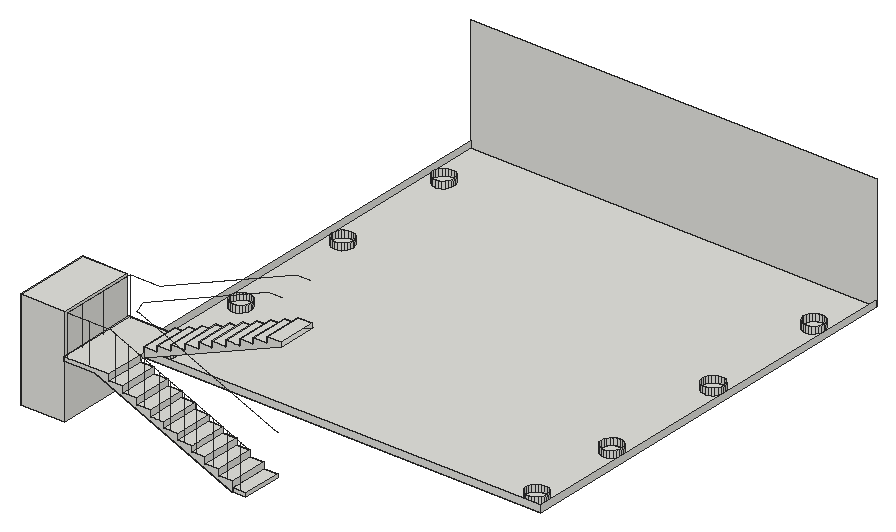
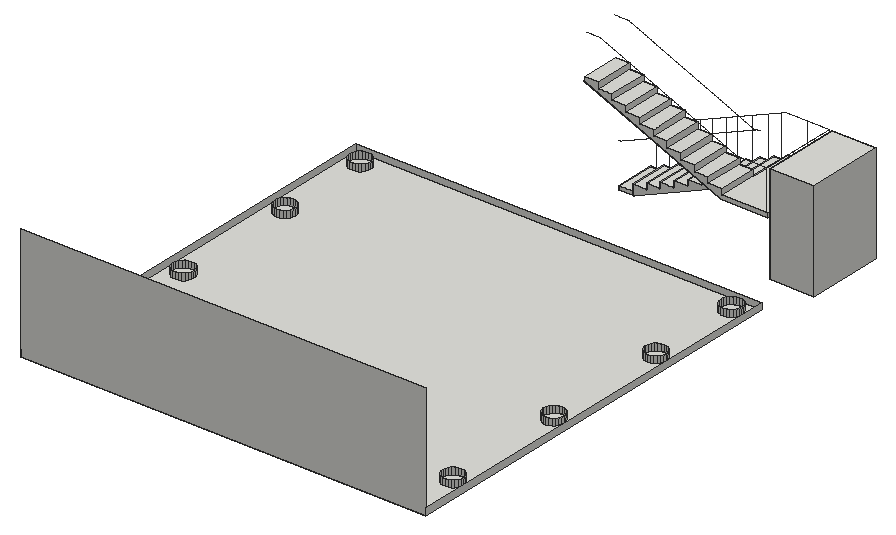
# SketchUp Ruby script. Lengths in millimetres.
U = 1.mm
M = Sketchup.active_model
def pt(a) = Geom::Point3d.new(a.map { |v| v * U })
def face(e, loops, mat)
  f = e.add_face(loops[0].map { |a| pt(a) })
  loops[1..].each { |l| e.add_face(l.map { |a| pt(a) }).erase! }
  f.material = f.back_material = mat if mat
  f
end
# faces: each face lists its corners as indices into pts; further lists are holes
def faces(e, pts, list, mat = nil) = list.each { |f| face(e, (f[0].is_a?(Array) ? f : [f]).map { |l| l.map { |i| pts[i] } }, mat) }
# xy, xz, yz: faces in a plane at the given z, y or x. An outline is a flat list of corners, or four numbers for a rectangle; further outlines are holes
def ring(l) = l.size == 4 ? [[l[0], l[1]], [l[2], l[1]], [l[2], l[3]], [l[0], l[3]]] : l.each_slice(2).to_a
def flat(e, list, mat, &to3) = list.each { |f| face(e, (f[0].is_a?(Array) ? f : [f]).map { |l| ring(l).map { |u, v| to3.(u, v) } }, mat) }
def xy(e, z, list, mat = nil) = flat(e, list, mat) { |x, y| [x, y, z] }
def xz(e, y, list, mat = nil) = flat(e, list, mat) { |x, z| [x, y, z] }
def yz(e, x, list, mat = nil) = flat(e, list, mat) { |y, z| [x, y, z] }
def lines(e, pts, list) = list.each { |a, b| e.add_line(pt(pts[a]), pt(pts[b])) }
# prism: a flat outline (further loops are holes) pulled along v
def prism(e, loops, v, mat = nil)
  f = face(e, loops, mat); d = Geom::Vector3d.new(v.map { |x| x * U })
  f.pushpull(f.normal.samedirection?(d) ? d.length : -d.length)
end
def box(e, o, s, mat = nil) = prism(e, [[o, [o[0] + s[0], o[1], o[2]], [o[0] + s[0], o[1] + s[1], o[2]], [o[0], o[1] + s[1], o[2]]]], [0, 0, s[2]], mat)
def at(x, y, z, deg = 0) = Geom::Transformation.translation(pt([x, y, z])) * Geom::Transformation.rotation(ORIGIN, Z_AXIS, deg.degrees)
def axes(o, x, y, z) = Geom::Transformation.new([*x, 0, *y, 0, *z, 0, *pt(o).to_a, 1])
def part(name) = M.definitions.add(name)
# library, detail: a bought-in or finely detailed component or shape, given as its bounding box
def library(name, o, s) = part(name).tap { |d| box(d.entities, o, s) }
def detail(e, o, s) = box(e.add_group.entities, o, s)
def put(e, d, t, mat = nil) = e.add_instance(d, t).tap { |i| i.material = mat if mat }
def group(e, t, mat = nil) = e.add_group.tap { |g| g.transformation = t; g.material = mat if mat }.entities
root = M.entities
c1 = part("Group55\#2")
p = [[13622.3,-331.8,4572],[13622.3,-282.6,4572],[13622.3,2717.8,6064.2],[13622.3,3668.7,6064.2],[15624.2,3668.7,6064.2],[15624.2,3017.8,6064.2],
  [15624.2,17.5,7556.5],[15624.2,-282.6,7556.5],[14524,-331.8,4572],[14524,-282.6,4572],[14524,2717.8,6064.2],[14524,2767,6064.2],
  [14722.5,2767,6189],[14722.5,17.5,7556.5],[14722.5,-282.6,7556.5]]
lines(c1.entities,p,[[0,1],[1,2],[2,3],[3,4],[4,5],[5,6],[6,7],[8,9],[9,10],[10,11],[11,12],[12,13],
  [13,14]])
c2 = part("Group54\#1")
xy(c2.entities,4472,[[13573.1,-282.6,14573.2,17.5],[13573.1,17.5,14573.2,41]])
xy(c2.entities,4572,[[13573.1,-282.6,14573.2,17.5]])
xy(c2.entities,4721.2,[[13573.1,17.5,14573.2,317.5]])
xy(c2.entities,4870.4,[[13573.1,317.5,14573.2,617.5]])
xy(c2.entities,5019.7,[[13573.1,617.5,14573.2,617.5,14573.3,917.6,13573.1,917.6]])
xy(c2.entities,5168.9,[[13573.1,917.6,14573.3,917.6,14573.2,1217.6,13573.1,1217.6]])
xy(c2.entities,5318.1,[[13573.1,1217.6,14573.2,1517.7]])
xy(c2.entities,5467.3,[[13573.1,1517.7,14573.2,1817.7]])
xy(c2.entities,5616.6,[[13573.1,1817.7,14573.2,2117.7]])
xy(c2.entities,5765.8,[[13573.1,2117.7,14573.2,2417.8]])
xy(c2.entities,5915,[[13573.1,2417.8,14573.2,2717.8]])
xy(c2.entities,5964.2,[[14673.3,2694.3,14673.3,2717.8,14573.2,2717.8,14573.2,3041.3,13573.1,3041.3,13573.1,3717.9,15673.4,3717.9,15673.4,2694.3]])
xy(c2.entities,6064.2,[[13573.1,2717.8,15673.4,3717.9]])
xy(c2.entities,6213.5,[[14673.3,2417.8,15673.4,2717.8]])
xy(c2.entities,6362.7,[[14673.3,2117.7,15673.4,2417.8]])
xy(c2.entities,6511.9,[[14673.3,1817.7,15673.4,2117.7]])
xy(c2.entities,6661.1,[[14673.3,1517.7,15673.4,1817.7]])
xy(c2.entities,6810.4,[[14673.3,1217.6,15673.4,1517.7]])
xy(c2.entities,6959.6,[[14673.3,917.6,15673.4,1217.6]])
xy(c2.entities,7108.8,[[14673.3,617.5,15673.4,917.6]])
xy(c2.entities,7258,[[14673.3,317.5,15673.4,617.5]])
xy(c2.entities,7407.3,[[14673.3,17.5,15673.4,317.5]])
xy(c2.entities,7556.5,[[14673.3,-282.6,15673.4,17.5]])
xz(c2.entities,-282.6,[[13573.1,4472,14573.2,4572]])
xz(c2.entities,17.5,[[13573.1,4472,14573.2,4572],[13573.1,4572,14573.2,4721.2],[14673.3,7407.3,15673.4,7556.5]])
xz(c2.entities,317.5,[[13573.1,4721.2,14573.2,4870.4],[14673.3,7258,15673.4,7407.3]])
xz(c2.entities,617.5,[[13573.1,4870.4,14573.2,5019.7],[14673.3,7108.8,15673.4,7258]])
xz(c2.entities,917.6,[[13573.1,5019.7,14573.3,5168.9],[14673.3,6959.6,15673.4,7108.8]])
xz(c2.entities,1217.6,[[13573.1,5168.9,14573.2,5318.1],[14673.3,6810.4,15673.4,6959.6]])
xz(c2.entities,1517.7,[[13573.1,5318.1,14573.2,5467.3],[14673.3,6661.1,15673.4,6810.4]])
xz(c2.entities,1817.7,[[13573.1,5467.3,14573.2,5616.6],[14673.3,6511.9,15673.4,6661.1]])
xz(c2.entities,2117.7,[[13573.1,5616.6,14573.2,5765.8],[14673.3,6362.7,15673.4,6511.9]])
xz(c2.entities,2417.8,[[13573.1,5765.8,14573.2,5915],[14673.3,6213.5,15673.4,6362.7]])
xz(c2.entities,2717.8,[[13573.1,5915,14573.2,6064.2],[14573.2,5964.2,14673.3,6064.2],[14673.3,6064.2,15673.4,6213.5]])
xz(c2.entities,3717.9,[[13573.1,5964.2,15673.4,6064.2]])
yz(c2.entities,13573.1,[[-282.6,4472,17.5,4572],[17.5,4472,17.5,4721.2,317.5,4721.2,317.5,4870.4,617.5,4870.4,617.5,5019.7,917.6,5019.7,917.6,5168.9,1217.6,5168.9,1217.6,5318.1,1517.7,5318.1,1517.7,5467.3,1817.7,5467.3,1817.7,5616.6,2117.7,5616.6,2117.7,5765.8,2417.8,5765.8,2417.8,5915,2717.8,5915,2717.8,6064.2,3717.9,6064.2,3717.9,5964.2,3041.3,5964.2,41,4472]])
yz(c2.entities,14573.2,[[-282.6,4472,17.5,4572]])
yz(c2.entities,14673.3,[[2694.3,5964.2,-306.1,7456.5,-282.6,7456.5,-282.6,7556.5,17.5,7556.5,17.5,7407.3,317.5,7407.3,317.5,7258,617.5,7258,617.5,7108.8,917.6,7108.8,917.6,6959.6,1217.6,6959.6,1217.6,6810.4,1517.7,6810.4,1517.7,6661.1,1817.7,6661.1,1817.7,6511.9,2117.7,6511.9,2117.7,6362.7,2417.8,6362.7,2417.8,6213.5,2717.8,6213.5,2717.8,5964.2]])
yz(c2.entities,15673.4,[[2694.3,5964.2,3717.9,5964.2,3717.9,6064.2,2717.8,6064.2,2717.8,6213.5,2417.8,6213.5,2417.8,6362.7,2117.7,6362.7,2117.7,6511.9,1817.7,6511.9,1817.7,6661.1,1517.7,6661.1,1517.7,6810.4,1217.6,6810.4,1217.6,6959.6,917.6,6959.6,917.6,7108.8,617.5,7108.8,617.5,7258,317.5,7258,317.5,7407.3,17.5,7407.3,17.5,7556.5,-282.6,7556.5,-282.6,7456.5,-306.1,7456.5]])
p = [[14573.2,3041.3,5964.2],[14573.2,2717.8,5964.2],[14573.2,2717.8,5915],[14573.2,2417.8,5915],[14573.2,2417.8,5765.8],[14573.2,2117.7,5765.8],
  [14573.2,2117.7,5616.6],[14573.2,1817.7,5616.6],[14573.2,1817.7,5467.3],[14573.2,1517.7,5467.3],[14573.2,1517.7,5318.1],[14573.2,1217.6,5318.1],
  [14573.2,1217.6,5168.9],[14573.3,917.6,5168.9],[14573.3,917.6,5019.7],[14573.2,617.5,5019.7],[14573.2,617.5,4870.4],[14573.2,317.5,4870.4],
  [14573.2,317.5,4721.2],[14573.2,17.5,4721.2],[14573.2,17.5,4572],[14573.2,17.5,4472],[14573.2,41,4472],[13573.1,41,4472],
  [13573.1,3041.3,5964.2],[15673.4,2694.3,5964.2],[15673.4,-306.1,7456.5],[14673.3,-306.1,7456.5],[14673.3,2694.3,5964.2],[13622.3,3193.3,7064.4],
  [13622.3,3193.3,6064.2],[13622.3,3668.7,7064.4],[13622.3,3668.7,6064.2],[15624.2,3668.7,7064.4],[15624.2,3668.7,6064.2],[14776.1,3668.7,7064.4],
  [14776.1,3668.7,6064.2],[14085.5,3668.7,7064.4],[14085.5,3668.7,6064.2],[13622.3,2628.2,7019.8],[13622.3,2628.2,5915],[13622.3,2338.2,6875.6],
  [13622.3,2338.2,5765.8],[13622.3,1987.6,6701.2],[13622.3,1987.6,5616.6],[13622.3,1654.5,6535.6],[13622.3,1654.5,5467.3],[13622.3,1115.8,6267.6],
  [13622.3,1115.8,5168.9],[13622.3,1403.5,6410.7],[13622.3,1403.5,5318.1],[13622.3,834.6,6127.8],[13622.3,834.6,5019.7],[13622.3,469.4,5946.1],
  [13622.3,469.4,4870.4],[13622.3,173.1,5798.7],[13622.3,173.1,4721.2],[13622.3,-122.5,5651.7],[13622.3,-122.5,4572]]
faces(c2.entities,p,[[0,1,2,3,4,5,6,7,8,9,10,11,12,13,14,15,16,17,18,19,20,21,22],[23,24,0,22],[25,26,27,28]])
lines(c2.entities,p,[[29,30],[31,32],[33,34],[35,36],[37,38],[39,40],[41,42],[43,44],[45,46],[47,48],[49,50],[51,52],
  [53,54],[55,56],[57,58]])
put(c2.entities,c1,at(0,0,1000.1))
xy(root,0,[[[720.2,4710,16417.4,20943.1],[15750.9,18372.1,15853.3,18390.3,15947.6,18434.3,16027.2,18501.2,16086.8,18586.5,16122.3,18684.3,16131.3,18787.9,16113.1,18890.3,16069.1,18984.6,16002.1,19064.2,15916.9,19123.8,15819.1,19159.3,15715.5,19168.3,15613.1,19150.1,15518.8,19106.1,15439.2,19039.1,15379.6,18953.9,15344.1,18856.1,15335.1,18752.5,15353.3,18650.1,15397.3,18555.8,15464.2,18476.2,15549.5,18416.6,15647.3,18381.1],[15768.9,8578.8,15871.3,8597,15965.5,8641,16045.1,8707.9,16104.7,8793.2,16140.2,8891,16149.2,8994.6,16131.1,9097,16087,9191.3,16020.1,9270.9,15934.8,9330.5,15837.1,9366,15733.4,9375,15631,9356.8,15536.8,9312.8,15457.1,9245.9,15397.6,9160.6,15362.1,9062.8,15353.1,8959.2,15371.2,8856.8,15415.3,8762.5,15482.2,8682.9,15567.5,8623.3,15665.2,8587.8],[1429.7,8578.8,1532.1,8597,1626.3,8641,1705.9,8707.9,1765.5,8793.2,1801,8891,1810,8994.6,1791.9,9097,1747.8,9191.3,1680.9,9270.9,1595.6,9330.5,1497.9,9366,1394.2,9375,1291.8,9356.8,1197.6,9312.8,1117.9,9245.9,1058.4,9160.6,1022.9,9062.8,1013.9,8959.2,1032,8856.8,1076.1,8762.5,1143,8682.9,1228.3,8623.3,1326,8587.8],[1429.7,18372.1,1532.1,18390.3,1626.3,18434.3,1705.9,18501.2,1765.5,18586.5,1801,18684.3,1810,18787.9,1791.9,18890.3,1747.8,18984.6,1680.9,19064.2,1595.6,19123.8,1497.9,19159.3,1394.2,19168.3,1291.8,19150.1,1197.6,19106.1,1117.9,19039.1,1058.4,18953.9,1022.9,18856.1,1013.9,18752.5,1032,18650.1,1076.1,18555.8,1143,18476.2,1228.3,18416.6,1326,18381.1],[1429.7,4921.2,1532.1,4939.4,1626.3,4983.4,1705.9,5050.3,1765.5,5135.6,1801,5233.4,1810,5337,1791.9,5439.4,1747.8,5533.7,1680.9,5613.3,1595.6,5672.9,1497.9,5708.4,1394.2,5717.4,1291.8,5699.2,1197.6,5655.2,1117.9,5588.3,1058.4,5503,1022.9,5405.2,1013.9,5301.6,1032,5199.2,1076.1,5104.9,1143,5025.3,1228.3,4965.7,1326,4930.2],[15787,4921.2,15889.4,4939.4,15983.7,4983.4,16063.3,5050.3,16122.9,5135.6,16158.4,5233.4,16167.4,5337,16149.2,5439.4,16105.2,5533.7,16038.3,5613.3,15953,5672.9,15855.2,5708.4,15751.6,5717.4,15649.2,5699.2,15554.9,5655.2,15475.3,5588.3,15415.7,5503,15380.2,5405.2,15371.2,5301.6,15389.4,5199.2,15433.4,5104.9,15500.3,5025.3,15585.6,4965.7,15683.4,4930.2],[15759.9,13504.8,15862.3,13523,15956.5,13567,16036.2,13634,16095.8,13719.2,16131.3,13817,16140.2,13920.6,16122.1,14023,16078.1,14117.3,16011.1,14196.9,15925.9,14256.5,15828.1,14292,15724.5,14301,15622,14282.8,15527.8,14238.8,15448.2,14171.9,15388.6,14086.6,15353.1,13988.8,15344.1,13885.2,15362.2,13782.8,15406.3,13688.5,15473.2,13608.9,15558.5,13549.3,15656.2,13513.8],[1429.7,13504.8,1532.1,13523,1626.3,13567,1705.9,13634,1765.5,13719.2,1801,13817,1810,13920.6,1791.9,14023,1747.8,14117.3,1680.9,14196.9,1595.6,14256.5,1497.9,14292,1394.2,14301,1291.8,14282.8,1197.6,14238.8,1117.9,14171.9,1058.4,14086.6,1022.9,13988.8,1013.9,13885.2,1032,13782.8,1076.1,13688.5,1143,13608.9,1228.3,13549.3,1326,13513.8]],[1429.7,4921.2,1326,4930.2,1228.3,4965.7,1143,5025.3,1076.1,5104.9,1032,5199.2,1013.9,5301.6,1022.9,5405.2,1058.4,5503,1117.9,5588.3,1197.6,5655.2,1291.8,5699.2,1394.2,5717.4,1497.9,5708.4,1595.6,5672.9,1680.9,5613.3,1747.8,5533.7,1791.9,5439.4,1810,5337,1801,5233.4,1765.5,5135.6,1705.9,5050.3,1626.3,4983.4,1532.1,4939.4],[15787,4921.2,15683.4,4930.2,15585.6,4965.7,15500.3,5025.3,15433.4,5104.9,15389.4,5199.2,15371.2,5301.6,15380.2,5405.2,15415.7,5503,15475.3,5588.3,15554.9,5655.2,15649.2,5699.2,15751.6,5717.4,15855.2,5708.4,15953,5672.9,16038.3,5613.3,16105.2,5533.7,16149.2,5439.4,16167.4,5337,16158.4,5233.4,16122.9,5135.6,16063.3,5050.3,15983.7,4983.4,15889.4,4939.4],[1429.7,8578.8,1326,8587.8,1228.3,8623.3,1143,8682.9,1076.1,8762.5,1032,8856.8,1013.9,8959.2,1022.9,9062.8,1058.4,9160.6,1117.9,9245.9,1197.6,9312.8,1291.8,9356.8,1394.2,9375,1497.9,9366,1595.6,9330.5,1680.9,9270.9,1747.8,9191.3,1791.9,9097,1810,8994.6,1801,8891,1765.5,8793.2,1705.9,8707.9,1626.3,8641,1532.1,8597],[15768.9,8578.8,15665.2,8587.8,15567.5,8623.3,15482.2,8682.9,15415.3,8762.5,15371.2,8856.8,15353.1,8959.2,15362.1,9062.8,15397.6,9160.6,15457.1,9245.9,15536.8,9312.8,15631,9356.8,15733.4,9375,15837.1,9366,15934.8,9330.5,16020.1,9270.9,16087,9191.3,16131.1,9097,16149.2,8994.6,16140.2,8891,16104.7,8793.2,16045.1,8707.9,15965.5,8641,15871.3,8597],
  [1429.7,13504.8,1326,13513.8,1228.3,13549.3,1143,13608.9,1076.1,13688.5,1032,13782.8,1013.9,13885.2,1022.9,13988.8,1058.4,14086.6,1117.9,14171.9,1197.6,14238.8,1291.8,14282.8,1394.2,14301,1497.9,14292,1595.6,14256.5,1680.9,14196.9,1747.8,14117.3,1791.9,14023,1810,13920.6,1801,13817,1765.5,13719.2,1705.9,13634,1626.3,13567,1532.1,13523],[15759.9,13504.8,15656.2,13513.8,15558.5,13549.3,15473.2,13608.9,15406.3,13688.5,15362.2,13782.8,15344.1,13885.2,15353.1,13988.8,15388.6,14086.6,15448.2,14171.9,15527.8,14238.8,15622,14282.8,15724.5,14301,15828.1,14292,15925.9,14256.5,16011.1,14196.9,16078.1,14117.3,16122.1,14023,16140.2,13920.6,16131.3,13817,16095.8,13719.2,16036.2,13634,15956.5,13567,15862.3,13523],[1429.7,18372.1,1326,18381.1,1228.3,18416.6,1143,18476.2,1076.1,18555.8,1032,18650.1,1013.9,18752.5,1022.9,18856.1,1058.4,18953.9,1117.9,19039.1,1197.6,19106.1,1291.8,19150.1,1394.2,19168.3,1497.9,19159.3,1595.6,19123.8,1680.9,19064.2,1747.8,18984.6,1791.9,18890.3,1810,18787.9,1801,18684.3,1765.5,18586.5,1705.9,18501.2,1626.3,18434.3,1532.1,18390.3],[15750.9,18372.1,15647.3,18381.1,15549.5,18416.6,15464.2,18476.2,15397.3,18555.8,15353.3,18650.1,15335.1,18752.5,15344.1,18856.1,15379.6,18953.9,15439.2,19039.1,15518.8,19106.1,15613.1,19150.1,15715.5,19168.3,15819.1,19159.3,15916.9,19123.8,16002.1,19064.2,16069.1,18984.6,16113.1,18890.3,16131.3,18787.9,16122.3,18684.3,16086.8,18586.5,16027.2,18501.2,15947.6,18434.3,15853.3,18390.3]])
xz(root,4710,[[720.2,0,16417.4,254]])
xz(root,20943.1,[[720.2,0,16417.4,4419.6]])
yz(root,720.2,[[4710,0,20943.1,254]])
yz(root,16417.4,[[4710,0,20943.1,254]])
p = [[1326,4930.2,0],[1429.7,4921.2,0],[1429.7,4921.2,254],[1326,4930.2,254],[1532.1,4939.4,0],[1532.1,4939.4,254],
  [15683.4,4930.2,0],[15787,4921.2,0],[15787,4921.2,254],[15683.4,4930.2,254],[15889.4,4939.4,0],[15889.4,4939.4,254],
  [1228.3,4965.7,0],[1228.3,4965.7,254],[15585.6,4965.7,0],[15585.6,4965.7,254],[1626.3,4983.4,0],[1626.3,4983.4,254],
  [15983.7,4983.4,0],[15983.7,4983.4,254],[1143,5025.3,0],[1143,5025.3,254],[15500.3,5025.3,0],[15500.3,5025.3,254],
  [1705.9,5050.3,0],[1705.9,5050.3,254],[16063.3,5050.3,0],[16063.3,5050.3,254],[1076.1,5104.9,0],[1076.1,5104.9,254],
  [15433.4,5104.9,0],[15433.4,5104.9,254],[1765.5,5135.6,0],[1765.5,5135.6,254],[16122.9,5135.6,0],[16122.9,5135.6,254],
  [1032,5199.2,0],[1032,5199.2,254],[15389.4,5199.2,0],[15389.4,5199.2,254],[1801,5233.4,0],[1801,5233.4,254],
  [16158.4,5233.4,0],[16158.4,5233.4,254],[1013.9,5301.6,0],[1013.9,5301.6,254],[15371.2,5301.6,0],[15371.2,5301.6,254],
  [1810,5337,0],[1810,5337,254],[16167.4,5337,0],[16167.4,5337,254],[1022.9,5405.2,0],[1022.9,5405.2,254],
  [15380.2,5405.2,0],[15380.2,5405.2,254],[1791.9,5439.4,0],[1791.9,5439.4,254],[16149.2,5439.4,0],[16149.2,5439.4,254],
  [1058.4,5503,0],[1058.4,5503,254],[15415.7,5503,0],[15415.7,5503,254],[1747.8,5533.7,0],[1747.8,5533.7,254],
  [16105.2,5533.7,0],[16105.2,5533.7,254],[1117.9,5588.3,0],[1117.9,5588.3,254],[15475.3,5588.3,0],[15475.3,5588.3,254],
  [1680.9,5613.3,0],[1680.9,5613.3,254],[16038.3,5613.3,0],[16038.3,5613.3,254],[1197.6,5655.2,0],[1197.6,5655.2,254],
  [15554.9,5655.2,0],[15554.9,5655.2,254],[1595.6,5672.9,0],[1595.6,5672.9,254],[15953,5672.9,0],[15953,5672.9,254],
  [1291.8,5699.2,0],[1291.8,5699.2,254],[15649.2,5699.2,0],[15649.2,5699.2,254],[1497.9,5708.4,0],[1497.9,5708.4,254],
  [15855.2,5708.4,0],[15855.2,5708.4,254],[1394.2,5717.4,0],[1394.2,5717.4,254],[15751.6,5717.4,0],[15751.6,5717.4,254],
  [1326,8587.8,0],[1429.7,8578.8,0],[1429.7,8578.8,254],[1326,8587.8,254],[1532.1,8597,0],[1532.1,8597,254],
  [15665.2,8587.8,0],[15768.9,8578.8,0],[15768.9,8578.8,254],[15665.2,8587.8,254],[15871.3,8597,0],[15871.3,8597,254],
  [1228.3,8623.3,0],[1228.3,8623.3,254],[15567.5,8623.3,0],[15567.5,8623.3,254],[1626.3,8641,0],[1626.3,8641,254],
  [15965.5,8641,0],[15965.5,8641,254],[1143,8682.9,0],[1143,8682.9,254],[15482.2,8682.9,0],[15482.2,8682.9,254],
  [1705.9,8707.9,0],[1705.9,8707.9,254],[16045.1,8707.9,0],[16045.1,8707.9,254],[1076.1,8762.5,0],[1076.1,8762.5,254],
  [15415.3,8762.5,0],[15415.3,8762.5,254],[1765.5,8793.2,0],[1765.5,8793.2,254],[16104.7,8793.2,0],[16104.7,8793.2,254],
  [1032,8856.8,0],[1032,8856.8,254],[15371.2,8856.8,0],[15371.2,8856.8,254],[1801,8891,0],[1801,8891,254],
  [16140.2,8891,0],[16140.2,8891,254],[1013.9,8959.2,0],[1013.9,8959.2,254],[15353.1,8959.2,0],[15353.1,8959.2,254],
  [1810,8994.6,0],[1810,8994.6,254],[16149.2,8994.6,0],[16149.2,8994.6,254],[1022.9,9062.8,0],[1022.9,9062.8,254],
  [15362.1,9062.8,0],[15362.1,9062.8,254],[1791.9,9097,0],[1791.9,9097,254],[16131.1,9097,0],[16131.1,9097,254],
  [1058.4,9160.6,0],[1058.4,9160.6,254],[15397.6,9160.6,0],[15397.6,9160.6,254],[1747.8,9191.3,0],[1747.8,9191.3,254],
  [16087,9191.3,0],[16087,9191.3,254],[1117.9,9245.9,0],[1117.9,9245.9,254],[15457.1,9245.9,0],[15457.1,9245.9,254],
  [1680.9,9270.9,0],[1680.9,9270.9,254],[16020.1,9270.9,0],[16020.1,9270.9,254],[1197.6,9312.8,0],[1197.6,9312.8,254],
  [15536.8,9312.8,0],[15536.8,9312.8,254],[1595.6,9330.5,0],[1595.6,9330.5,254],[15934.8,9330.5,0],[15934.8,9330.5,254],
  [1291.8,9356.8,0],[1291.8,9356.8,254],[15631,9356.8,0],[15631,9356.8,254],[1497.9,9366,0],[1497.9,9366,254],
  [15837.1,9366,0],[15837.1,9366,254],[1394.2,9375,0],[1394.2,9375,254],[15733.4,9375,0],[15733.4,9375,254],
  [1326,13513.8,0],[1429.7,13504.8,0],[1429.7,13504.8,254],[1326,13513.8,254],[1532.1,13523,0],[1532.1,13523,254],
  [15656.2,13513.8,0],[15759.9,13504.8,0],[15759.9,13504.8,254],[15656.2,13513.8,254],[15862.3,13523,0],[15862.3,13523,254],
  [1228.3,13549.3,0],[1228.3,13549.3,254],[15558.5,13549.3,0],[15558.5,13549.3,254],[1626.3,13567,0],[1626.3,13567,254],
  [15956.5,13567,0],[15956.5,13567,254],[1143,13608.9,0],[1143,13608.9,254],[15473.2,13608.9,0],[15473.2,13608.9,254],
  [1705.9,13634,0],[1705.9,13634,254],[16036.2,13634,0],[16036.2,13634,254],[1076.1,13688.5,0],[1076.1,13688.5,254],
  [15406.3,13688.5,0],[15406.3,13688.5,254],[1765.5,13719.2,0],[1765.5,13719.2,254],[16095.8,13719.2,0],[16095.8,13719.2,254],
  [1032,13782.8,0],[1032,13782.8,254],[15362.2,13782.8,0],[15362.2,13782.8,254],[1801,13817,0],[1801,13817,254],
  [16131.3,13817,0],[16131.3,13817,254],[1013.9,13885.2,0],[1013.9,13885.2,254],[15344.1,13885.2,0],[15344.1,13885.2,254],
  [1810,13920.6,0],[1810,13920.6,254],[16140.2,13920.6,0],[16140.2,13920.6,254],[1022.9,13988.8,0],[1022.9,13988.8,254],
  [15353.1,13988.8,0],[15353.1,13988.8,254],[1791.9,14023,0],[1791.9,14023,254],[16122.1,14023,0],[16122.1,14023,254],
  [1058.4,14086.6,0],[1058.4,14086.6,254],[15388.6,14086.6,0],[15388.6,14086.6,254],[1747.8,14117.3,0],[1747.8,14117.3,254],
  [16078.1,14117.3,0],[16078.1,14117.3,254],[1117.9,14171.9,0],[1117.9,14171.9,254],[15448.2,14171.9,0],[15448.2,14171.9,254],
  [1680.9,14196.9,0],[1680.9,14196.9,254],[16011.1,14196.9,0],[16011.1,14196.9,254],[1197.6,14238.8,0],[1197.6,14238.8,254],
  [15527.8,14238.8,0],[15527.8,14238.8,254],[1595.6,14256.5,0],[1595.6,14256.5,254],[15925.9,14256.5,0],[15925.9,14256.5,254],
  [1291.8,14282.8,0],[1291.8,14282.8,254],[15622,14282.8,0],[15622,14282.8,254],[1497.9,14292,0],[1497.9,14292,254],
  [15828.1,14292,0],[15828.1,14292,254],[1394.2,14301,0],[1394.2,14301,254],[15724.5,14301,0],[15724.5,14301,254],
  [1326,18381.1,0],[1429.7,18372.1,0],[1429.7,18372.1,254],[1326,18381.1,254],[1532.1,18390.3,0],[1532.1,18390.3,254],
  [15647.3,18381.1,0],[15750.9,18372.1,0],[15750.9,18372.1,254],[15647.3,18381.1,254],[15853.3,18390.3,0],[15853.3,18390.3,254],
  [1228.3,18416.6,0],[1228.3,18416.6,254],[15549.5,18416.6,0],[15549.5,18416.6,254],[1626.3,18434.3,0],[1626.3,18434.3,254],
  [15947.6,18434.3,0],[15947.6,18434.3,254],[1143,18476.2,0],[1143,18476.2,254],[15464.2,18476.2,0],[15464.2,18476.2,254],
  [1705.9,18501.2,0],[1705.9,18501.2,254],[16027.2,18501.2,0],[16027.2,18501.2,254],[1076.1,18555.8,0],[1076.1,18555.8,254],
  [15397.3,18555.8,0],[15397.3,18555.8,254],[1765.5,18586.5,0],[1765.5,18586.5,254],[16086.8,18586.5,0],[16086.8,18586.5,254],
  [1032,18650.1,0],[1032,18650.1,254],[15353.3,18650.1,0],[15353.3,18650.1,254],[1801,18684.3,0],[1801,18684.3,254],
  [16122.3,18684.3,0],[16122.3,18684.3,254],[1013.9,18752.5,0],[1013.9,18752.5,254],[15335.1,18752.5,0],[15335.1,18752.5,254],
  [1810,18787.9,0],[1810,18787.9,254],[16131.3,18787.9,0],[16131.3,18787.9,254],[1022.9,18856.1,0],[1022.9,18856.1,254],
  [15344.1,18856.1,0],[15344.1,18856.1,254],[1791.9,18890.3,0],[1791.9,18890.3,254],[16113.1,18890.3,0],[16113.1,18890.3,254],
  [1058.4,18953.9,0],[1058.4,18953.9,254],[15379.6,18953.9,0],[15379.6,18953.9,254],[1747.8,18984.6,0],[1747.8,18984.6,254],
  [16069.1,18984.6,0],[16069.1,18984.6,254],[1117.9,19039.1,0],[1117.9,19039.1,254],[15439.2,19039.1,0],[15439.2,19039.1,254],
  [1680.9,19064.2,0],[1680.9,19064.2,254],[16002.1,19064.2,0],[16002.1,19064.2,254],[1197.6,19106.1,0],[1197.6,19106.1,254],
  [15518.8,19106.1,0],[15518.8,19106.1,254],[1595.6,19123.8,0],[1595.6,19123.8,254],[15916.9,19123.8,0],[15916.9,19123.8,254],
  [1291.8,19150.1,0],[1291.8,19150.1,254],[15613.1,19150.1,0],[15613.1,19150.1,254],[1497.9,19159.3,0],[1497.9,19159.3,254],
  [15819.1,19159.3,0],[15819.1,19159.3,254],[1394.2,19168.3,0],[1394.2,19168.3,254],[15715.5,19168.3,0],[15715.5,19168.3,254]]
faces(root,p,[[0,1,2,3],[1,4,5,2],[6,7,8,9],[7,10,11,8],[12,0,3,13],[14,6,9,15],[4,16,17,5],[10,18,19,11],
  [20,12,13,21],[22,14,15,23],[16,24,25,17],[18,26,27,19],[28,20,21,29],[30,22,23,31],[24,32,33,25],[26,34,35,27],
  [36,28,29,37],[38,30,31,39],[32,40,41,33],[34,42,43,35],[44,36,37,45],[46,38,39,47],[40,48,49,41],[42,50,51,43],
  [52,44,45,53],[54,46,47,55],[48,56,57,49],[50,58,59,51],[60,52,53,61],[62,54,55,63],[56,64,65,57],[58,66,67,59],
  [68,60,61,69],[70,62,63,71],[64,72,73,65],[66,74,75,67],[76,68,69,77],[78,70,71,79],[72,80,81,73],[74,82,83,75],
  [84,76,77,85],[86,78,79,87],[80,88,89,81],[82,90,91,83],[92,84,85,93],[94,86,87,95],[88,92,93,89],[90,94,95,91],
  [96,97,98,99],[97,100,101,98],[102,103,104,105],[103,106,107,104],[108,96,99,109],[110,102,105,111],[100,112,113,101],[106,114,115,107],
  [116,108,109,117],[118,110,111,119],[112,120,121,113],[114,122,123,115],[124,116,117,125],[126,118,119,127],[120,128,129,121],[122,130,131,123],
  [132,124,125,133],[134,126,127,135],[128,136,137,129],[130,138,139,131],[140,132,133,141],[142,134,135,143],[136,144,145,137],[138,146,147,139],
  [148,140,141,149],[150,142,143,151],[144,152,153,145],[146,154,155,147],[156,148,149,157],[158,150,151,159],[152,160,161,153],[154,162,163,155],
  [164,156,157,165],[166,158,159,167],[160,168,169,161],[162,170,171,163],[172,164,165,173],[174,166,167,175],[168,176,177,169],[170,178,179,171],
  [180,172,173,181],[182,174,175,183],[176,184,185,177],[178,186,187,179],[188,180,181,189],[190,182,183,191],[184,188,189,185],[186,190,191,187],
  [192,193,194,195],[193,196,197,194],[198,199,200,201],[199,202,203,200],[204,192,195,205],[206,198,201,207],[196,208,209,197],[202,210,211,203],
  [212,204,205,213],[214,206,207,215],[208,216,217,209],[210,218,219,211],[220,212,213,221],[222,214,215,223],[216,224,225,217],[218,226,227,219],
  [228,220,221,229],[230,222,223,231],[224,232,233,225],[226,234,235,227],[236,228,229,237],[238,230,231,239],[232,240,241,233],[234,242,243,235],
  [244,236,237,245],[246,238,239,247],[240,248,249,241],[242,250,251,243],[252,244,245,253],[254,246,247,255],[248,256,257,249],[250,258,259,251],
  [260,252,253,261],[262,254,255,263],[256,264,265,257],[258,266,267,259],[268,260,261,269],[270,262,263,271],[264,272,273,265],[266,274,275,267],
  [276,268,269,277],[278,270,271,279],[272,280,281,273],[274,282,283,275],[284,276,277,285],[286,278,279,287],[280,284,285,281],[282,286,287,283],
  [288,289,290,291],[289,292,293,290],[294,295,296,297],[295,298,299,296],[300,288,291,301],[302,294,297,303],[292,304,305,293],[298,306,307,299],
  [308,300,301,309],[310,302,303,311],[304,312,313,305],[306,314,315,307],[316,308,309,317],[318,310,311,319],[312,320,321,313],[314,322,323,315],
  [324,316,317,325],[326,318,319,327],[320,328,329,321],[322,330,331,323],[332,324,325,333],[334,326,327,335],[328,336,337,329],[330,338,339,331],
  [340,332,333,341],[342,334,335,343],[336,344,345,337],[338,346,347,339],[348,340,341,349],[350,342,343,351],[344,352,353,345],[346,354,355,347],
  [356,348,349,357],[358,350,351,359],[352,360,361,353],[354,362,363,355],[364,356,357,365],[366,358,359,367],[360,368,369,361],[362,370,371,363],
  [372,364,365,373],[374,366,367,375],[368,376,377,369],[370,378,379,371],[380,372,373,381],[382,374,375,383],[376,380,381,377],[378,382,383,379]])
put(root,c2,axes([8298.7,-20477.8,-6828.5],[0,1.5087,0],[-1.76518,0,0],[0,0,1.5087]))
g1 = group(root,at(0,74.2,0))
box(g1,[0,0,0],[1711.6,3020.2,3829.5])
